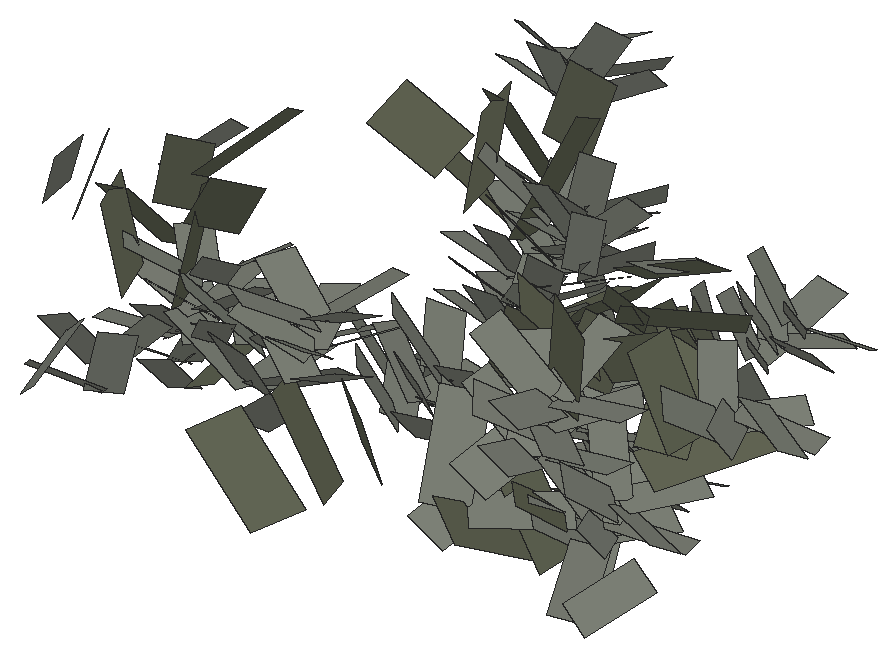
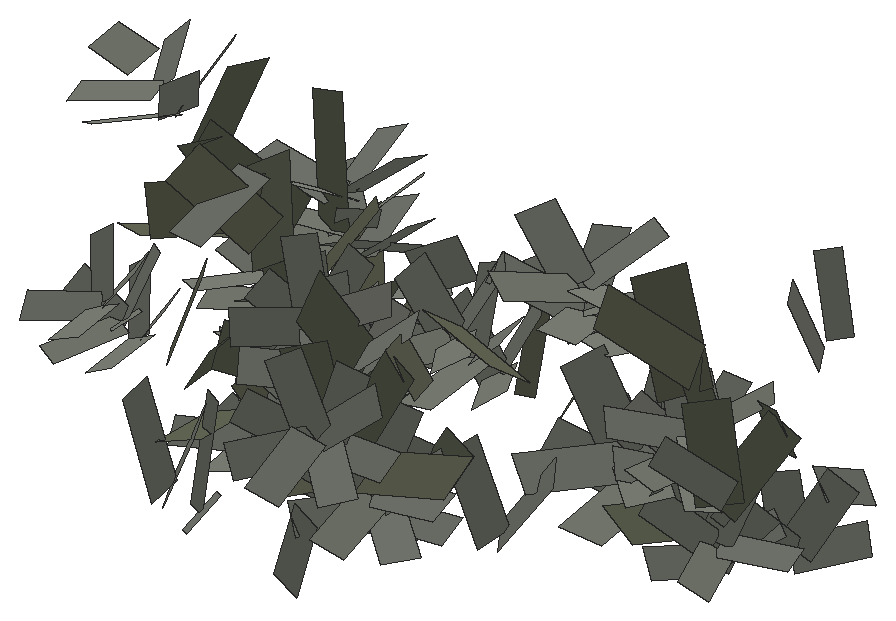
# SketchUp Ruby script. Lengths in inches.
U = 1.inch
M = Sketchup.active_model
def pt(a) = Geom::Point3d.new(a.map { |v| v * U })
def face(e, loops, mat)
  f = e.add_face(loops[0].map { |a| pt(a) })
  loops[1..].each { |l| e.add_face(l.map { |a| pt(a) }).erase! }
  f.material = f.back_material = mat if mat
  f
end
# faces: each face lists its corners as indices into pts; further lists are holes
def faces(e, pts, list, mat = nil) = list.each { |f| face(e, (f[0].is_a?(Array) ? f : [f]).map { |l| l.map { |i| pts[i] } }, mat) }
# xy, xz, yz: faces in a plane at the given z, y or x. An outline is a flat list of corners, or four numbers for a rectangle; further outlines are holes
def ring(l) = l.size == 4 ? [[l[0], l[1]], [l[2], l[1]], [l[2], l[3]], [l[0], l[3]]] : l.each_slice(2).to_a
def flat(e, list, mat, &to3) = list.each { |f| face(e, (f[0].is_a?(Array) ? f : [f]).map { |l| ring(l).map { |u, v| to3.(u, v) } }, mat) }
def xy(e, z, list, mat = nil) = flat(e, list, mat) { |x, y| [x, y, z] }
def xz(e, y, list, mat = nil) = flat(e, list, mat) { |x, z| [x, y, z] }
def yz(e, x, list, mat = nil) = flat(e, list, mat) { |y, z| [x, y, z] }
def lines(e, pts, list) = list.each { |a, b| e.add_line(pt(pts[a]), pt(pts[b])) }
# prism: a flat outline (further loops are holes) pulled along v
def prism(e, loops, v, mat = nil)
  f = face(e, loops, mat); d = Geom::Vector3d.new(v.map { |x| x * U })
  f.pushpull(f.normal.samedirection?(d) ? d.length : -d.length)
end
def box(e, o, s, mat = nil) = prism(e, [[o, [o[0] + s[0], o[1], o[2]], [o[0] + s[0], o[1] + s[1], o[2]], [o[0], o[1] + s[1], o[2]]]], [0, 0, s[2]], mat)
def at(x, y, z, deg = 0) = Geom::Transformation.translation(pt([x, y, z])) * Geom::Transformation.rotation(ORIGIN, Z_AXIS, deg.degrees)
def axes(o, x, y, z) = Geom::Transformation.new([*x, 0, *y, 0, *z, 0, *pt(o).to_a, 1])
def part(name) = M.definitions.add(name)
# library, detail: a bought-in or finely detailed component or shape, given as its bounding box
def library(name, o, s) = part(name).tap { |d| box(d.entities, o, s) }
def detail(e, o, s) = box(e.add_group.entities, o, s)
def put(e, d, t, mat = nil) = e.add_instance(d, t).tap { |i| i.material = mat if mat }
def group(e, t, mat = nil) = e.add_group.tap { |g| g.transformation = t; g.material = mat if mat }.entities
root = M.entities
M.materials.add("viburnumblaasdfas0df1w06d").color = [98, 102, 84]
M.materials.add("viburnumbladsadfasdfad0w122").color = [125, 129, 119]
c1 = part("Component\#314")
p = [[0.14,0,0],[2.58,0.05,0.25],[2.44,5.11,2.64],[0,5.05,2.39]]
faces(c1.entities,p,[[0,1,2,3]],"viburnumblaasdfas0df1w06d")
c2 = part("viburnumblad1\#2")
put(c2.entities,c1,axes([-37.25,6.23,19.31],[75.98784,0,0],[0,65.50676,0],[0,0,75.98784]))
c3 = part("Component\#315")
p = [[0.25,0,0],[2.05,0.01,0.35],[1.81,4.2,1.66],[0,4.19,1.3125]]
faces(c3.entities,p,[[0,1,2,3]],"viburnumbladsadfasdfad0w122")
c4 = part("viburnumblad2")
put(c4.entities,c3,axes([-19.23,-4.49,-32.18],[83.35428,0,0],[0,79.38502,0],[0,0,83.35428]))
put(root,c2,axes([2216.9,270.47,29.54],[-0.011,0.0051,0.00655],[-0.00551,-0.01483,0.0023],[0.00681,-0.00067,0.01196]))
put(root,c4,axes([2205.93,270.18,36.3125],[-0.01209,-0.0034,-0.0003],[0.00332,-0.01209,0.00349],[-0.00129,0.00365,0.01095]))
put(root,c4,axes([2205.76,269.54,37.9],[-0.01088,0.00599,-0.0016],[-0.00628,-0.01045,0.00254],[-0.00013,0.00352,0.01104]))
put(root,c4,axes([2219.11,270.46,37.76],[-0.01207,0.00042,0.00346],[-0.00034,-0.01255,0.00035],[0.00347,0.00024,0.01207]))
put(root,c2,axes([2204.65,266.57,27.99],[0.00623,0.01349,0.00121],[-0.0157,0.00724,0.00014],[-0.00044,-0.00098,0.01352]))
put(root,c4,axes([2190.32,267.16,30.32],[0.00946,-0.00383,0.00571],[0.00246,0.01108,0.00318],[-0.00637,-0.00125,0.00808]))
put(root,c4,axes([2190.61,270.14,39.96],[0.00021,-0.01046,-0.0046],[0.00792,-0.00325,0.00774],[-0.00831,-0.0033,0.00712]))
put(root,c4,axes([2214.1,266.34,33.47],[0.00902,0.01086,-0.00673],[-0.00719,0.01113,0.00831],[0.01056,-0.0017,0.01141]))
put(root,c4,axes([2218.1,270.6,34.8125],[-0.0126,0.00044,0.00361],[-0.00031,-0.0113,0.00032],[0.00347,0.00024,0.01207]))
put(root,c4,axes([2205.46,270.44,34.83],[-0.00597,-0.01037,0.00113],[0.01154,-0.00613,0.0032],[-0.00222,0.00293,0.01099]))
put(root,c2,axes([2207.0625,268.11,29.67],[-0.00512,0.01258,-0.00225],[-0.01225,-0.00318,0.00944],[0.00707,0.00483,0.00942]))
put(root,c2,axes([2217.31,271.55,31.83],[-0.01089,-0.0066,0.00527],[0.00777,-0.0139,-0.00135],[0.00514,0.00164,0.01268]))
put(root,c4,axes([2221.26,267.54,30.01],[0.00733,0.00034,-0.00907],[0.00348,0.00978,0.00299],[0.00808,-0.00497,0.00546]))
put(root,c4,axes([2220.3,267.6,29.09],[0.00746,0.0085,-0.0048],[-0.00195,0.00645,0.00799],[0.00881,-0.00455,0.00477]))
put(root,c4,axes([2214.24,268.09,33.36],[0.00842,-0.01125,-0.00685],[0.01063,0.01127,-0.00543],[0.00843,-0.00165,0.01307]))
put(root,c2,axes([2208.35,270.08,30.46],[-0.01166,0.00571,0.00452],[-0.00151,-0.01177,0.01017],[0.0071,0.00732,0.00793]))
put(root,c4,axes([2205.3,268.85,36.45],[-0.0033,0.01188,-0.00196],[-0.01112,-0.00285,0.00099],[0.00058,0.00262,0.01122]))
put(root,c4,axes([2218.33,270.01,36.22],[-0.008,0.00913,0.00324],[-0.00789,-0.00792,0.00285],[0.00448,-0.00024,0.01173]))
put(root,c4,axes([2218.32,271.48,36.4],[-0.00907,-0.00853,0.00165],[0.00877,-0.00968,-0.00184],[0.0024,-0.00017,0.01233]))
put(root,c4,axes([2205.61,271.09,37.66],[-0.00622,-0.0108,0.00117],[0.01069,-0.00568,0.00296],[-0.00222,0.00293,0.01099]))
put(root,c4,axes([2228.56,271.66,39.8],[-0.00908,-0.00254,0.00688],[0.00302,-0.01141,-0.00024],[0.00679,0.00165,0.00837]))
put(root,c4,axes([2221.14,271.65,31.72],[-0.00974,-0.00261,0.006],[0.00353,-0.01123,0.00072],[0.00551,0.00254,0.00899]))
put(root,c4,axes([2220.21,270.97,30.78],[-0.00853,0.00601,0.00433],[-0.00446,-0.01051,0.00545],[0.00645,0.00235,0.00846]))
put(root,c4,axes([2212.86,267.17,32],[0.01184,-0.00027,-0.00922],[0.00172,0.01671,0.00172],[0.00948,-0.00223,0.01224]))
put(root,c4,axes([2227.48,271.09,38.95],[-0.00764,0.00611,0.00552],[-0.0043,-0.01063,0.00535],[0.00765,0.00146,0.00773]))
put(root,c4,axes([2221.76,270.9,33.03],[-0.00889,0.00626,0.00451],[-0.00413,-0.00973,0.00504],[0.00645,0.00235,0.00846]))
put(root,c4,axes([2215.02,267.45,35.29],[0.01234,-0.00028,-0.00961],[0.00159,0.01547,0.00159],[0.00948,-0.00223,0.01224]))
put(root,c4,axes([2217.81,269.59,38.03],[0.00076,0.01249,0.00112],[-0.01157,0.00026,0.0049],[0.00485,-0.00133,0.01151]))
put(root,c4,axes([2204.4,268.72,35.14],[0.00564,0.00974,-0.00221],[-0.01091,0.00622,-0.00021],[0.00111,0.00263,0.01119]))
put(root,c4,axes([2192.31,271.05,29.6],[-0.00614,0.00518,-0.0082],[-0.00794,-0.00715,0.00088],[-0.00475,0.00709,0.00648]))
put(root,c4,axes([2190.82,270.47,38.47],[0.00662,-0.00815,0.00069],[0.00514,0.00494,0.00894],[-0.00725,-0.00529,0.00709]))
put(root,c4,axes([2217.05,269.79,35.125],[0.00022,0.01156,-0.00012],[-0.01157,0.00026,0.0049],[0.0049,0.00003,0.01157]))
put(root,c4,axes([2229.24,272.28,41],[-0.00489,-0.00995,0.00397],[0.00876,-0.00628,-0.0047],[0.00608,0.00102,0.00892]))
put(root,c2,axes([2217.91,270.14,29.08],[0.00107,0.01287,0.00071],[-0.01171,0.00034,0.00907],[0.0079,-0.00141,0.00892]))
put(root,c4,axes([2221.62,272.39,32.95],[-0.00489,-0.00995,0.00397],[0.00954,-0.00607,-0.00338],[0.00477,0.0019,0.00949]))
put(root,c4,axes([2218.31,271.78,38.125],[-0.00076,-0.01249,-0.00112],[0.01239,-0.00058,-0.00197],[0.0019,-0.00123,0.01236]))
put(root,c4,axes([2204.76,270.96,36.15],[0.0033,-0.01188,0.00196],[0.01189,0.00365,0.00167],[-0.00236,0.00179,0.01115]))
put(root,c4,axes([2217.17,271.85,35.17],[-0.00073,-0.01199,-0.00108],[0.01339,-0.00063,-0.00213],[0.0019,-0.00123,0.01236]))
put(root,c4,axes([2220.49,270.59,32.1875],[-0.00283,0.01146,0.00038],[-0.0094,-0.00257,0.00741],[0.00704,0.00146,0.00821]))
put(root,c2,axes([2224.92,270.49,37.5],[0.00184,0.01273,0.00122],[-0.0105,0.00029,0.01027],[0.00896,-0.0024,0.00784]))
put(root,c4,axes([2191.86,272.39,30.3],[-0.01,-0.00241,-0.00568],[-0.00201,-0.00892,0.00667],[-0.00557,0.00722,0.00577]))
put(root,c4,axes([2192.36,272.18,28.86],[-0.008,-0.00859,0.00017],[0.00566,-0.00462,0.00938],[-0.00647,0.00667,0.0055]))
put(root,c4,axes([2204.18,269.37,37.82],[0.00622,0.0108,-0.00117],[-0.01091,0.00622,-0.00021],[0.00044,0.00147,0.01138]))
put(root,c4,axes([2208.94,272.68,32.23],[-0.00734,-0.00647,0.00686],[0.01022,-0.00834,0.00267],[0.00284,0.00722,0.00872]))
put(root,c2,axes([2218.16,271.53,36.08],[-0.01355,0.00411,0.00465],[0.00135,-0.01078,0.01345],[0.00609,0.01091,0.00813]))
put(root,c4,axes([2208.95,271.34,33.07],[-0.00945,0.00892,-0.00145],[-0.0064,-0.00533,0.00736],[0.00487,0.007,0.00802]))
put(root,c4,axes([2200.49,273.08,31.1],[-0.01458,-0.00076,0.00047],[0.00121,-0.01217,0.00796],[0.00032,0.00837,0.01162]))
put(root,c4,axes([2209.86,272.8,33.51],[-0.01181,0.00128,0.00407],[0.00154,-0.01046,0.00743],[0.00382,0.0075,0.00815]))
put(root,c4,axes([2199.99,273.2,29.27],[-0.0086,-0.00967,0.00326],[0.01109,-0.00774,0.00569],[-0.00192,0.00675,0.01234]))
put(root,c4,axes([2219.47,269.75,29.39],[0.00909,0.00791,-0.00471],[-0.00403,0.00937,0.00796],[0.00828,-0.00412,0.00905]))
put(root,c4,axes([2196.97,273.35,33.79],[-0.01133,0.00035,-0.0015],[-0.0009,-0.01068,0.0043],[-0.00126,0.00434,0.0105]))
put(root,c4,axes([2203.76,269.71,36.26],[0.01209,0.0034,0.0003],[-0.00342,0.01218,-0.00058],[-0.00049,0.00075,0.01143]))
put(root,c4,axes([2216.64,270.07,36.74],[0.00907,0.00853,-0.00165],[-0.0076,0.009,0.00473],[0.00435,-0.00239,0.01154]))
put(root,c4,axes([2196.89,273.79,32.32],[-0.00757,-0.0073,-0.00011],[0.00727,-0.00761,0.00446],[-0.00317,0.00314,0.01053]))
put(root,c4,axes([2216.97,271.64,36.82],[0.008,-0.00913,-0.00324],[0.00942,0.00831,-0.00017],[0.00227,-0.00232,0.01214]))
put(root,c4,axes([2227.64,272.66,40.45],[0.00217,-0.01153,-0.00126],[0.00998,0.00257,-0.00587],[0.00594,-0.00007,0.00905]))
put(root,c4,axes([2204.03,270.92,37.58],[0.01088,-0.00599,0.0016],[0.00606,0.01099,0.00021],[-0.00165,0.00089,0.01133]))
put(root,c4,axes([2220.1,272.64,32.21],[0.00283,-0.01146,-0.00038],[0.01049,0.00275,-0.00491],[0.00467,0.00082,0.00968]))
put(root,c4,axes([2218.96,270.77,31.57],[0.0051,0.01038,-0.00415],[-0.00729,0.00572,0.00502],[0.00694,0.00038,0.0084]))
put(root,c4,axes([2226.33,270.89,39.87],[0.0051,0.01038,-0.00415],[-0.00633,0.00571,0.00604],[0.00802,-0.00053,0.00751]))
put(root,c4,axes([2199.9,273.07,33.125],[-0.01112,0.00864,-0.0042],[-0.00937,-0.00881,0.00635],[0.00161,0.00797,0.01181]))
put(root,c4,axes([2220.49,270.83,33.79],[0.00489,0.00995,-0.00397],[-0.0081,0.00635,0.00558],[0.00694,0.00038,0.0084]))
put(root,c4,axes([2196.19,273.04,35.3],[-0.00749,0.00804,-0.00315],[-0.00863,-0.00712,0.00235],[-0.00031,0.00392,0.01074]))
put(root,c4,axes([2210.16,272.87,35.19],[-0.00905,0.00854,-0.00139],[-0.00711,-0.00593,0.00818],[0.00487,0.007,0.00802]))
put(root,c4,axes([2210.29,274.18,34.36],[-0.00765,-0.00673,0.00714],[0.00947,-0.00772,0.00247],[0.00284,0.00722,0.00872]))
put(root,c4,axes([2217.01,270.92,38.4],[0.01207,-0.00042,-0.00346],[0.00117,0.01224,0.00258],[0.00328,-0.0028,0.0118]))
put(root,c4,axes([2196.53,274.4,34.96],[-0.00853,-0.00755,0.00102],[0.00727,-0.00761,0.00446],[-0.00226,0.00398,0.01048]))
put(root,c2,axes([2193.4,271.36,34.14],[0.00699,0.00088,0.01038],[-0.00621,0.01278,0.0031],[-0.00893,-0.00592,0.00652]))
put(root,c4,axes([2195.03,274.39,29.09],[-0.00996,-0.0034,-0.00378],[0.00101,-0.00837,0.00457],[-0.00471,0.00422,0.00764]))
put(root,c2,axes([2222.75,270.89,36.74],[0.00961,0.00746,-0.00443],[-0.00604,0.01187,0.00656],[0.0068,-0.00274,0.00947]))
put(root,c4,axes([2200.07,274.71,32.32],[-0.0095,-0.00972,0.00486],[0.01109,-0.00774,0.00569],[-0.0009,0.00784,0.01189]))
put(root,c4,axes([2219.39,271.23,32.74],[0.00974,0.00261,-0.006],[-0.00192,0.01057,0.00135],[0.0062,-0.00026,0.0089]))
put(root,c4,axes([2199.07,272.01,31.64],[-0.00115,0.01298,-0.0064],[-0.01441,0.00008,0.00199],[0.00223,0.00688,0.01234]))
put(root,c4,axes([2209.04,271.92,34.35],[-0.00099,0.0108,-0.00603],[-0.01031,0.00186,0.00471],[0.00538,0.00602,0.00839]))
put(root,c4,axes([2218.83,272.03,31.61],[0.00761,-0.00572,-0.00506],[0.00557,0.01001,-0.00285],[0.00619,-0.00075,0.00889]))
put(root,c4,axes([2208.92,273.84,33.31],[0.00099,-0.0108,0.00603],[0.0122,-0.00051,-0.00294],[0.0025,0.00634,0.00938]))
put(root,c4,axes([2191.27,273.22,29.27],[-0.00132,-0.00974,0.00592],[0.00922,0.00313,0.00644],[-0.00695,0.00574,0.0058]))
put(root,c4,axes([2226.27,272.16,39.97],[0.00664,-0.00572,-0.00612],[0.00571,0.0099,-0.00294],[0.00728,-0.00165,0.00803]))
put(root,c2,axes([2196.22,274.92,36.53],[-0.00965,-0.00928,0.0022],[0.01068,-0.00958,0.00645],[-0.00246,0.00545,0.01217]))
put(root,c4,axes([2195.75,272.55,33.86],[0.00073,0.01102,-0.00295],[-0.01141,0.00071,-0.00016],[0.00003,0.00295,0.01104]))
put(root,c4,axes([2220.34,272.31,33.7],[0.00889,-0.00626,-0.00451],[0.00557,0.01001,-0.00285],[0.00526,-0.00007,0.00943]))
put(root,c4,axes([2194.45,274.37,30.15],[-0.00794,0.00459,-0.00546],[-0.00557,-0.00804,0.00123],[-0.00382,0.00415,0.0081]))
put(root,c2,axes([2195.05,273.39,33.1875],[0.00608,-0.01136,0.00423],[0.00607,0.0078,0.01224],[-0.01094,-0.0031,0.0074]))
put(root,c4,axes([2207.7,271.67,33.5],[0.00649,0.00565,-0.00743],[-0.0085,0.00924,-0.00029],[0.00584,0.00584,0.00823]))
put(root,c4,axes([2194.01,275.34,31.1],[-0.00954,-0.00326,-0.00362],[0.00113,-0.0093,0.00507],[-0.00471,0.00422,0.00764]))
put(root,c4,axes([2195.92,274.48,33.32],[-0.00073,-0.01102,0.00295],[0.01017,0.00002,0.00259],[-0.00273,0.00304,0.01068]))
put(root,c4,axes([2198.92,274.28,30.47],[0.00115,-0.01298,0.0064],[0.01333,0.00146,0.00097],[-0.00132,0.00669,0.01246]))
put(root,c4,axes([2194.16,275.49,29.65],[-0.00555,-0.00919,0.00035],[0.0077,-0.00439,0.00674],[-0.00547,0.00359,0.00747]))
put(root,c2,axes([2221.17,272.34,35.06],[0.01127,-0.00662,-0.00498],[0.00702,0.01432,-0.0031],[0.00548,-0.00011,0.01154]))
put(root,c2,axes([2217.87,274.39,37.12],[-0.00474,-0.00612,0.0114],[0.01476,-0.00511,0.0034],[0.00234,0.01154,0.00716]))
put(root,c4,axes([2195.49,272.54,32.36],[0.00819,0.00724,-0.00098],[-0.00821,0.00902,-0.00193],[-0.00044,0.00202,0.01125]))
put(root,c4,axes([2193.15,274.29,31.03],[-0.00169,0.00975,-0.0041],[-0.01002,-0.00286,-0.00259],[-0.00334,0.00343,0.00858]))
put(root,c4,axes([2195.7,273.95,32.04],[0.00782,-0.00839,0.00329],[0.00747,0.00707,0.00029],[-0.00239,0.00208,0.01099]))
put(root,c4,axes([2207.78,273.15,34.18],[0.01181,-0.00128,-0.00407],[-0.00051,0.0116,-0.00495],[0.00406,0.00486,0.00962]))
put(root,c4,axes([2214.95,275.73,31.57],[-0.00706,0.00732,-0.0001],[-0.00736,-0.00703,0.00431],[0.00303,0.00306,0.01018]))
put(root,c4,axes([2215.61,276.67,32.53],[-0.01066,0.00071,0.00285],[0.00002,-0.00983,0.00251],[0.00294,0.00264,0.01033]))
put(root,c4,axes([2194.8,273.32,35.05],[0.00853,0.00755,-0.00102],[-0.0076,0.00835,-0.00179],[-0.00044,0.00202,0.01125]))
put(root,c4,axes([2215.1,276.89,31.29],[-0.00812,-0.00757,0.00318],[0.00684,-0.00722,0.00028],[0.00201,0.00231,0.01062]))
put(root,c2,axes([2195.59,272.83,29.32],[0.01125,-0.00276,0.00479],[0.00395,0.01395,-0.00123],[-0.00436,0.00225,0.01154]))
put(root,c4,axes([2208.67,273.26,35.57],[0.00765,0.00673,-0.00714],[-0.0085,0.00924,-0.00029],[0.00504,0.00514,0.00906]))
put(root,c4,axes([2208.8,274.58,34.73],[0.00905,-0.00854,0.00139],[0.00807,0.00744,-0.006],[0.00301,0.00536,0.00976]))
put(root,c2,axes([2216.04,276.38,35.63],[-0.00897,0.00933,0.00213],[-0.00926,-0.01033,0.00624],[0.00527,0.00238,0.01177]))
put(root,c4,axes([2194.99,273.52,33.48],[0.01133,-0.00035,0.0015],[0.00059,0.01187,-0.00167],[-0.00144,0.00165,0.01122]))
put(root,c4,axes([2195.13,274.69,34.71],[0.00749,-0.00804,0.00315],[0.0083,0.00786,0.00032],[-0.00239,0.00208,0.01099]))
put(root,c4,axes([2215.54,276.08,34.12],[-0.0073,0.00825,0.00099],[-0.00736,-0.00703,0.00431],[0.00384,0.00219,0.01013]))
put(root,c2,axes([2192.51,276.75,33.79],[-0.01098,0.00138,-0.00403],[-0.00375,-0.01153,0.00597],[-0.00261,0.00614,0.00861]))
put(root,c4,axes([2198.0625,273.26,33.05],[0.0095,0.00972,-0.00486],[-0.01098,0.00941,-0.00264],[0.00181,0.00573,0.01291]))
put(root,c4,axes([2197.91,273.07,31.09],[0.01458,0.00076,-0.00047],[-0.00114,0.0144,-0.00508],[0.00059,0.00521,0.01318]))
put(root,c4,axes([2215.82,277.43,33.88],[-0.00778,-0.00725,0.00304],[0.0076,-0.00802,0.00031],[0.00201,0.00231,0.01062]))
put(root,c4,axes([2193.14,276.11,30.41],[0.00169,-0.00975,0.0041],[0.00892,0.0036,0.00459],[-0.00566,0.00263,0.0077]))
put(root,c2,axes([2214.02,276.98,28.66],[-0.00267,-0.01088,0.00464],[0.01349,-0.00382,-0.00119],[0.00218,0.00422,0.01116]))
put(root,c4,axes([2198.23,274.89,32.24],[0.01112,-0.00864,0.0042],[0.00948,0.01048,-0.0033],[-0.0007,0.0056,0.01299]))
put(root,c2,axes([2194.29,275.54,38.4375],[0.00364,-0.01074,0.00535],[0.01254,0.00622,0.00396],[-0.00521,0.00362,0.01082]))
put(root,c2,axes([2216.64,278.24,37.48],[-0.01039,-0.00352,0.00517],[0.00601,-0.01213,0.00383],[0.0035,0.00504,0.01046]))
put(root,c4,axes([2193.0625,275.22,29.22],[0.00794,-0.00459,0.00546],[0.00496,0.0095,0.00066],[-0.00518,0.00191,0.00818]))
put(root,c4,axes([2214.52,275.65,32.99],[0.00034,0.01095,-0.00145],[-0.01033,0.00087,0.00416],[0.0042,0.00122,0.01016]))
put(root,c4,axes([2214.69,277.57,32.68],[-0.00034,-0.01095,0.00145],[0.01148,-0.00057,-0.00162],[0.0016,0.00139,0.01085]))
put(root,c4,axes([2192.28,275.0625,30.34],[0.00954,0.00326,0.00362],[-0.00223,0.01005,-0.00307],[-0.00429,0.00184,0.00864]))
put(root,c2,axes([2214.56,277.51,32.4],[-0.01099,-0.00588,0.00409],[0.00754,-0.00587,0.01184],[-0.00299,0.01058,0.00715]))
put(root,c2,axes([2217.08,275.92,39.02],[0.00672,-0.00769,0.00925],[0.01396,0.00492,-0.00605],[0.00006,0.01062,0.00878]))
put(root,c2,axes([2191.375,278.41,34.48],[-0.00937,-0.00701,0.00111],[0.00657,-0.00694,0.00934],[-0.00422,0.00731,0.00713]))
put(root,c4,axes([2216.59,278.37,28.98],[-0.00889,0.00537,0.00033],[-0.00425,-0.00744,0.00652],[0.00347,0.00529,0.00723]))
put(root,c4,axes([2213.74,277.09,31.6],[0.00701,-0.00792,-0.00095],[0.00872,0.00794,-0.00187],[0.00195,0.00042,0.01087]))
put(root,c4,axes([2217.19,279.36,29.72],[-0.00943,-0.00164,0.00397],[0.00349,-0.00863,0.00444],[0.00255,0.00548,0.00745]))
put(root,c4,axes([2214.23,276.41,34.45],[0.00778,0.00725,-0.00304],[-0.00689,0.00834,0.00227],[0.00379,0.0003,0.01038]))
put(root,c4,axes([2203.53,279.68,28.99],[-0.01014,-0.00518,0.00703],[0.00849,-0.00835,0.00609],[0.00203,0.00907,0.00962]))
put(root,c4,axes([2216.34,279.43,28.5625],[-0.00444,-0.00768,0.00528],[0.00919,-0.00479,0.00064],[0.00185,0.00501,0.00791]))
put(root,c4,axes([2214.5,277.75,34.2],[0.0073,-0.00825,-0.00099],[0.00807,0.00735,-0.00173],[0.00195,0.00042,0.01087]))
put(root,c4,axes([2213.75,276.84,33.06],[0.01066,-0.00071,-0.00285],[0.00069,0.01103,-0.00015],[0.00286,-0.00003,0.01068]))
put(root,c4,axes([2203.08,278.47,30.07],[-0.00818,0.0094,-0.00487],[-0.00969,-0.00417,0.00823],[0.00426,0.00856,0.00935]))
put(root,c2,axes([2216,279.35,39.34],[-0.00272,-0.01048,0.00546],[0.01366,-0.00332,0.00044],[0.00096,0.00539,0.01082]))
put(root,c4,axes([2216.45,278.52,30.39],[-0.00315,0.00923,-0.0035],[-0.009,-0.00109,0.00491],[0.00408,0.00455,0.00739]))
put(root,c4,axes([2217.16,277.4,42.04],[0.01174,-0.00224,-0.0016],[0.00091,0.0107,-0.00829],[0.00274,0.00736,0.0098]))
put(root,c2,axes([2207.91,280.27,28.37],[-0.01202,0.00402,-0.00269],[-0.00561,-0.01134,0.00795],[0.00019,0.00723,0.00942]))
put(root,c4,axes([2215.51,278.09,29.47],[0.00444,0.00768,-0.00528],[-0.00777,0.00538,0.00119],[0.00402,0.0037,0.00783]))
put(root,c4,axes([2189.34,279.66,35.8],[0.00099,-0.00884,0.00502],[0.00961,0.00407,0.00487],[-0.00586,0.00398,0.00703]))
put(root,c4,axes([2216.18,280.19,29.65],[0.00315,-0.00923,0.0035],[0.00972,0.00216,-0.00297],[0.00178,0.00415,0.00836]))
put(root,c4,axes([2211.74,281.61,37.51],[-0.00788,-0.0064,0.00067],[0.00477,-0.00497,0.00864],[-0.00511,0.00701,0.00686]))
put(root,c2,axes([2212.6,279.1,33.32],[0.00085,-0.00676,0.01003],[0.01236,0.00601,0.00299],[-0.00572,0.00864,0.0063]))
put(root,c4,axes([2211.42,281.81,38.95],[-0.01012,-0.0002,-0.00445],[-0.00314,-0.00766,0.00749],[-0.00319,0.00804,0.00689]))
put(root,c4,axes([2208.82,282.66,35.09],[-0.00994,-0.00547,0.00222],[0.00636,-0.00933,0.00551],[-0.00082,0.00596,0.01103]))
put(root,c2,axes([2219.41,281.06,33.65],[-0.00677,0.00906,0.00107],[-0.00671,-0.00636,0.00903],[0.00707,0.00408,0.0069]))
put(root,c4,axes([2215.4375,279.35,30.3125],[0.00943,0.00164,-0.00397],[-0.00277,0.00969,-0.0025],[0.00332,0.00323,0.0083]))
put(root,c4,axes([2209.03,282.42,36.75],[-0.01209,0.00339,-0.00041],[-0.00309,-0.0102,0.00689],[0.00151,0.00666,0.01054]))
put(root,c2,axes([2207.21,282.31,29.2],[-0.01137,-0.00525,0.00325],[0.00699,-0.00886,0.00961],[-0.00151,0.00884,0.00798]))
put(root,c2,axes([2217.8125,279.96,32.98],[0.00134,0.01062,-0.0039],[-0.01115,0.00362,0.00577],[0.00594,0.00252,0.00833]))
put(root,c4,axes([2220.63,283.03,34.93],[-0.00855,-0.00095,0.00486],[0.00394,-0.00929,0.00471],[0.00385,0.00566,0.0068]))
put(root,c4,axes([2210.29,282.15,40.13],[-0.00525,0.00588,-0.00776],[-0.00943,-0.00525,0.0024],[-0.00241,0.00775,0.0075]))
put(root,c2,axes([2204.18,280.28,40.14],[0.00447,0.01094,0.00709],[-0.01215,0.00867,-0.00572],[-0.00776,-0.00379,0.01074]))
put(root,c4,axes([2210.17,281.14,38.99],[0.0027,0.00851,-0.00652],[-0.01047,0.00066,-0.00347],[-0.00228,0.00703,0.00822]))
put(root,c4,axes([2206.51,283.28,31.7],[-0.01201,-0.00131,-0.00224],[-0.00042,-0.0083,0.00649],[-0.00262,0.00705,0.00788]))
put(root,c2,axes([2207.51,281.35,29.77],[0.00221,-0.01095,0.00807],[0.01572,0.00285,-0.00044],[-0.00114,0.008,0.01116]))
put(root,c4,axes([2209.03,283.85,37.84],[-0.01083,-0.00527,0.00359],[0.00636,-0.00933,0.00551],[0.00035,0.00657,0.01071]))
put(root,c4,axes([2210.85,283.21,39.42],[-0.00906,-0.00616,0.00146],[0.00477,-0.00497,0.00864],[-0.00416,0.00772,0.00674]))
put(root,c4,axes([2210.29,280.54,37.65],[0.0087,0.00591,-0.0014],[-0.00609,0.00723,-0.0073],[-0.00288,0.00629,0.00863]))
put(root,c2,axes([2211.15,279.57,34.99],[0.00897,-0.0006,0.00814],[0.00562,0.01175,-0.00532],[-0.00657,0.00665,0.00773]))
put(root,c4,axes([2221.21,283,36.11],[-0.00853,0.00582,0.00111],[-0.0037,-0.00695,0.00724],[0.00473,0.00542,0.00649]))
put(root,c4,axes([2210.6875,282.62,37.83],[-0.0027,-0.00851,0.00652],[0.00882,0.00097,0.00492],[-0.00475,0.00698,0.00714]))
put(root,c4,axes([2210.73,281.64,36.89],[0.00548,-0.00614,0.0081],[0.00771,0.00628,-0.00046],[-0.00462,0.00625,0.00786]))
put(root,c4,axes([2208.37,282.57,38.52],[-0.00627,0.01006,-0.00416],[-0.01061,-0.00457,0.00494],[0.00244,0.00598,0.01078]))
put(root,c4,axes([2221.96,283.99,36.73],[-0.00891,-0.00099,0.00506],[0.00365,-0.0086,0.00436],[0.00385,0.00566,0.0068]))
put(root,c2,axes([2215.93,279.88,31.5],[0.01113,0.00289,-0.00438],[-0.00454,0.01328,-0.00273],[0.00348,0.00335,0.01016]))
put(root,c4,axes([2208.15,283.82,36.125],[-0.00322,-0.01084,0.00548],[0.01114,-0.00248,0.00163],[-0.00036,0.00575,0.01116]))
put(root,c4,axes([2220.95,284.06,35.68],[-0.00407,-0.00723,0.00605],[0.00898,-0.00522,-0.00021],[0.0032,0.00525,0.00736]))
put(root,c4,axes([2220.04,282.19,35.74],[-0.00329,0.00963,-0.00365],[-0.00749,-0.00039,0.00532],[0.00532,0.00466,0.00661]))
put(root,c4,axes([2206.06,283.61,32.91],[-0.00804,0.00619,-0.0059],[-0.0078,-0.0066,0.00358],[-0.00163,0.0068,0.00829]))
put(root,c4,axes([2205.5,282.5625,32],[0.00025,0.00856,-0.00655],[-0.01174,-0.00053,-0.00107],[-0.00121,0.00703,0.00818]))
put(root,c4,axes([2207.56,283.12,34.88],[0.00655,-0.0105,0.00435],[0.00979,0.0053,-0.00197],[-0.0002,0.0047,0.01165]))
put(root,c4,axes([2207.54,281.94,37.125],[0.00322,0.01084,-0.00548],[-0.01186,0.00402,0.00097],[0.00259,0.00493,0.01126]))
put(root,c4,axes([2205.97,284.78,32.18],[-0.00824,-0.00797,0.00286],[0.00803,-0.0057,0.00726],[-0.00361,0.00659,0.00792]))
put(root,c4,axes([2206.01,284.9,33.79],[-0.01151,-0.00126,-0.00215],[-0.00046,-0.00922,0.00721],[-0.00262,0.00705,0.00788]))
put(root,c4,axes([2209.67,281.85,38.08],[0.01012,0.0002,0.00445],[0.00236,0.00977,-0.0058],[-0.00385,0.00596,0.00848]))
put(root,c2,axes([2206.92,282.91,36.31],[0.00407,-0.01295,0.00616],[0.01043,0.00846,0.01089],[-0.01117,0.00115,0.0098]))
put(root,c2,axes([2204.8,281.42,37.92],[0.00927,0.00064,0.01018],[-0.00266,0.0157,0.00144],[-0.00994,-0.00253,0.00921]))
put(root,c4,axes([2221.27,283.21,37.51],[-0.00315,0.00923,-0.0035],[-0.00832,-0.00043,0.00591],[0.00532,0.00466,0.00661]))
put(root,c4,axes([2216.14,284.45,29.02],[-0.01262,0.00712,0.00249],[-0.00199,-0.00788,0.01243],[0.00728,0.01023,0.00765]))
put(root,c4,axes([2209.09,282.31,39.44],[0.00906,0.00616,-0.00146],[-0.00564,0.00669,-0.00676],[-0.00288,0.00629,0.00863]))
put(root,c4,axes([2205.58,284.14,30.9],[-0.00014,-0.00961,0.00594],[0.01198,0.00212,0.00345],[-0.00404,0.00568,0.00838]))
put(root,c4,axes([2207.02,281.76,35.54],[0.01039,0.00506,-0.00344],[-0.00658,0.01149,-0.00298],[0.00188,0.00411,0.01172]))
put(root,c2,axes([2206.72,281.52,32.2],[0.0119,-0.00534,0.00444],[0.00766,0.01326,-0.00459],[-0.00215,0.00555,0.01243]))
put(root,c4,axes([2209.64,283.37,38.72],[0.00525,-0.00588,0.00776],[0.00856,0.00697,-0.00051],[-0.00462,0.00625,0.00786]))
put(root,c4,axes([2220.1875,282.79,36.73],[0.00407,0.00723,-0.00605],[-0.00729,0.00582,0.00182],[0.00528,0.00383,0.00709]))
put(root,c4,axes([2220.98,284.87,36.74],[0.00315,-0.00923,0.0035],[0.00936,0.00154,-0.00413],[0.00315,0.00442,0.00785]))
put(root,c4,axes([2219.21,282.94,35.83],[0.00769,0.00057,-0.00539],[-0.00261,0.00972,-0.00258],[0.00555,0.0035,0.00706]))
put(root,c4,axes([2204.81,284.05,34.02],[0.00014,0.01001,-0.00619],[-0.01174,-0.00053,-0.00107],[-0.00123,0.00599,0.0089]))
put(root,c4,axes([2207.6,284.5,37.67],[0.00627,-0.01006,0.00416],[0.01088,0.00589,-0.00218],[-0.0002,0.0047,0.01165]))
put(root,c4,axes([2206.9375,283.12,36.6],[0.01209,-0.00339,0.00041],[0.0035,0.01198,-0.00427],[0.00073,0.00402,0.01188]))
put(root,c4,axes([2216.85,286.35,29.57],[-0.01093,-0.00132,0.00974],[0.00771,-0.01018,0.00728],[0.00609,0.01052,0.00826]))
put(root,c4,axes([2219.76,284.11,36.25],[0.00853,-0.00582,-0.00111],[0.00461,0.00781,-0.00517],[0.00374,0.00366,0.00797]))
put(root,c4,axes([2204.43,283.45,32.64],[0.00824,0.00797,-0.00286],[-0.00838,0.00693,-0.00484],[-0.00165,0.00508,0.00936]))
put(root,c4,axes([2206.9375,283.22,38.35],[0.01083,0.00527,-0.00359],[-0.00609,0.01064,-0.00276],[0.00188,0.00411,0.01172]))
put(root,c4,axes([2205.18,285.85,32.99],[-0.00014,-0.01001,0.00619],[0.0111,0.00196,0.00319],[-0.00404,0.00568,0.00838]))
put(root,c4,axes([2220.29,284.09,37.51],[0.00891,0.00099,-0.00506],[-0.00261,0.00972,-0.00258],[0.00462,0.00341,0.00766]))
put(root,c4,axes([2204.67,284.74,31.89],[0.00804,-0.00619,0.0059],[0.00785,0.00862,-0.00178],[-0.00364,0.00486,0.00899]))
put(root,c2,axes([2204.56,284.95,35.3],[-0.00083,0.01216,-0.00686],[-0.01618,-0.00142,-0.00053],[-0.00101,0.00652,0.01095]))
put(root,c4,axes([2216.23,285.39,31.02],[-0.00691,0.01139,-0.00621],[-0.01,-0.00019,0.01077],[0.00826,0.00929,0.00783]))
put(root,c4,axes([2214.63,284.5,30.14],[0.00284,0.00899,-0.01128],[-0.01167,0.00819,0.00358],[0.00847,0.00827,0.00872]))
put(root,c2,axes([2205.23,287.26,36.56],[-0.01186,0.00394,-0.00337],[-0.00604,-0.00999,0.00917],[0.00026,0.00862,0.00831]))
put(root,c4,axes([2203.98,284.99,33.22],[0.01151,0.00126,0.00215],[-0.00018,0.01065,-0.00509],[-0.00265,0.00461,0.00939]))
put(root,c4,axes([2208.26,288.125,29.55],[-0.01122,0.00147,-0.00326],[-0.00368,-0.004,0.01025],[0.00008,0.01052,0.00323]))
put(root,c2,axes([2204.58,289.44,37.09],[-0.01156,-0.00444,0.00366],[0.00659,-0.0076,0.0107],[-0.00137,0.01006,0.00666]))
put(root,c4,axes([2203.87,290.8125,39.41],[-0.01201,-0.00131,-0.00224],[-0.00075,-0.00731,0.00743],[-0.00252,0.0083,0.00677]))
put(root,c4,axes([2202.84,290.16,39.77],[0.00059,0.00756,-0.00753],[-0.01174,-0.00037,-0.00119],[-0.00112,0.00828,0.00709]))
put(root,c4,axes([2203.42,291.33,40.55],[-0.00777,0.00552,-0.00673],[-0.00804,-0.00584,0.00423],[-0.00155,0.00808,0.00722]))
put(root,c4,axes([2203.37,292.39,39.67],[-0.0085,-0.0073,0.00369],[0.00776,-0.00483,0.008],[-0.00353,0.00786,0.00685]))
put(root,c4,axes([2202.99,291.57,38.49],[-0.0005,-0.0087,0.00708],[0.01199,0.0023,0.00332],[-0.00399,0.00704,0.00741]))
put(root,c4,axes([2201.79,291.17,40.26],[0.0085,0.0073,-0.00369],[-0.00811,0.00643,-0.0058],[-0.00164,0.00652,0.00849]))
put(root,c4,axes([2202.08,292.35,39.375],[0.00777,-0.00552,0.00673],[0.00812,0.00813,-0.00272],[-0.00362,0.0063,0.00812]))
put(root,c4,axes([2201.38,292.8125,40.63],[0.01151,0.00126,0.00215],[0.0002,0.00988,-0.00637],[-0.00265,0.00609,0.00857]))
